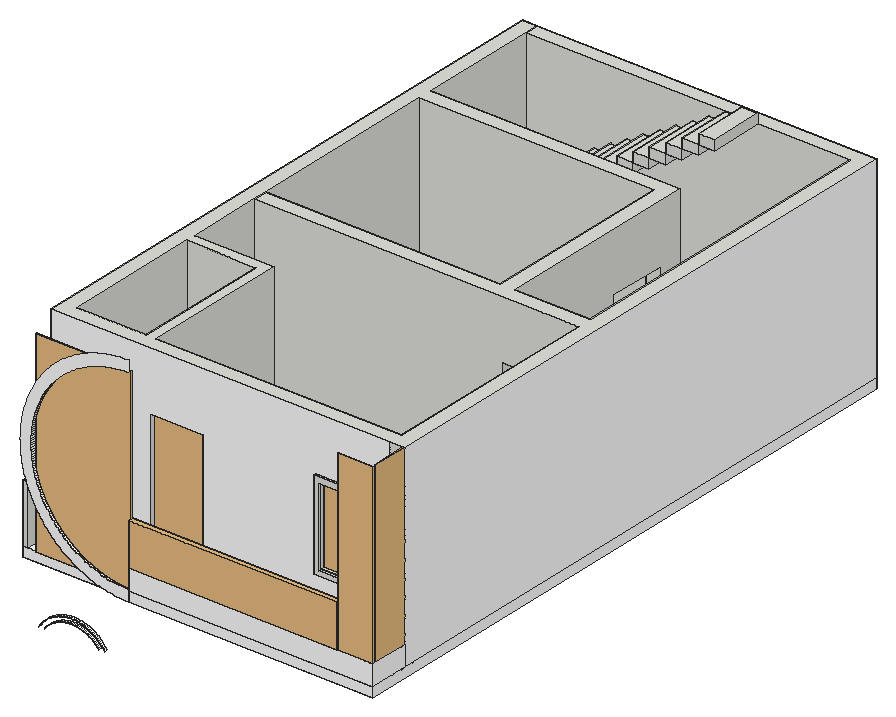
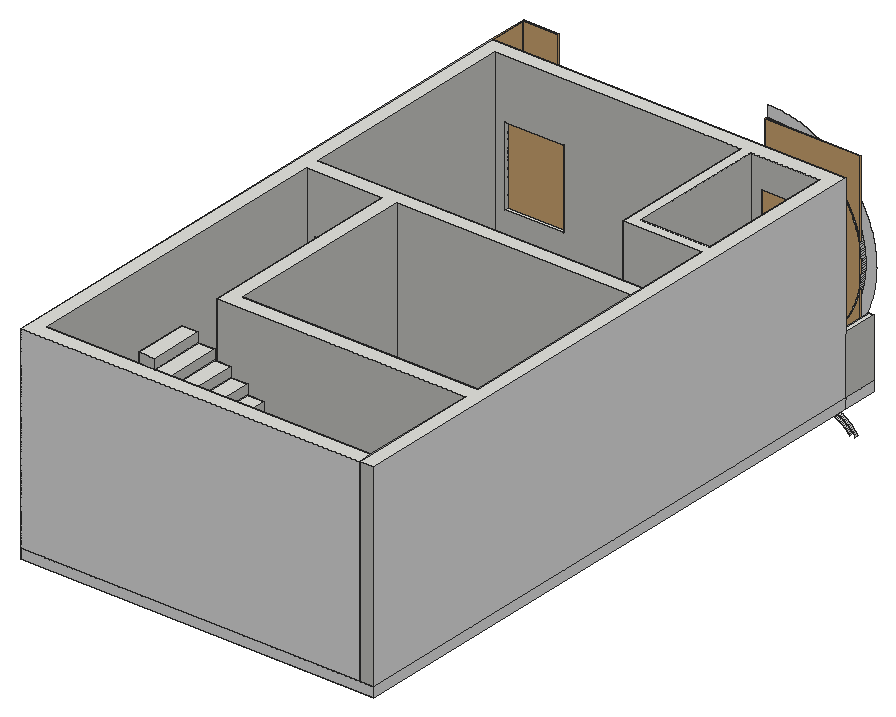
# SketchUp Ruby script. Lengths in inches.
U = 1.inch
M = Sketchup.active_model
def pt(a) = Geom::Point3d.new(a.map { |v| v * U })
def face(e, loops, mat)
  f = e.add_face(loops[0].map { |a| pt(a) })
  loops[1..].each { |l| e.add_face(l.map { |a| pt(a) }).erase! }
  f.material = f.back_material = mat if mat
  f
end
# faces: each face lists its corners as indices into pts; further lists are holes
def faces(e, pts, list, mat = nil) = list.each { |f| face(e, (f[0].is_a?(Array) ? f : [f]).map { |l| l.map { |i| pts[i] } }, mat) }
# xy, xz, yz: faces in a plane at the given z, y or x. An outline is a flat list of corners, or four numbers for a rectangle; further outlines are holes
def ring(l) = l.size == 4 ? [[l[0], l[1]], [l[2], l[1]], [l[2], l[3]], [l[0], l[3]]] : l.each_slice(2).to_a
def flat(e, list, mat, &to3) = list.each { |f| face(e, (f[0].is_a?(Array) ? f : [f]).map { |l| ring(l).map { |u, v| to3.(u, v) } }, mat) }
def xy(e, z, list, mat = nil) = flat(e, list, mat) { |x, y| [x, y, z] }
def xz(e, y, list, mat = nil) = flat(e, list, mat) { |x, z| [x, y, z] }
def yz(e, x, list, mat = nil) = flat(e, list, mat) { |y, z| [x, y, z] }
def lines(e, pts, list) = list.each { |a, b| e.add_line(pt(pts[a]), pt(pts[b])) }
# prism: a flat outline (further loops are holes) pulled along v
def prism(e, loops, v, mat = nil)
  f = face(e, loops, mat); d = Geom::Vector3d.new(v.map { |x| x * U })
  f.pushpull(f.normal.samedirection?(d) ? d.length : -d.length)
end
def box(e, o, s, mat = nil) = prism(e, [[o, [o[0] + s[0], o[1], o[2]], [o[0] + s[0], o[1] + s[1], o[2]], [o[0], o[1] + s[1], o[2]]]], [0, 0, s[2]], mat)
def at(x, y, z, deg = 0) = Geom::Transformation.translation(pt([x, y, z])) * Geom::Transformation.rotation(ORIGIN, Z_AXIS, deg.degrees)
def axes(o, x, y, z) = Geom::Transformation.new([*x, 0, *y, 0, *z, 0, *pt(o).to_a, 1])
def part(name) = M.definitions.add(name)
# library, detail: a bought-in or finely detailed component or shape, given as its bounding box
def library(name, o, s) = part(name).tap { |d| box(d.entities, o, s) }
def detail(e, o, s) = box(e.add_group.entities, o, s)
def put(e, d, t, mat = nil) = e.add_instance(d, t).tap { |i| i.material = mat if mat }
def group(e, t, mat = nil) = e.add_group.tap { |g| g.transformation = t; g.material = mat if mat }.entities
root = M.entities
M.materials.add("Leather White 002 15.0cm").color = [255, 255, 255]
M.materials.add("Manhattan Creative Coating ML 1016B 24.75cm").color = [255, 255, 255]
M.materials.add("Napura - nsi3013 29.32cm").color = [255, 255, 255]
M.materials.add("Wood 012 27.21cm").color = [255, 255, 255]
c1 = library("Door 243 053",[-21.6,-2.79,-0.07],[43.2,5.58,82.64])
c2 = part("Stair tread")
box(c2.entities,[0,0,0],[10,33,6])
c3 = part("Stair landing")
box(c3.entities,[-32,0,0],[42,72,6])
c4 = part("Group\#2")
put(c4.entities,c2,at(82,39,90))
put(c4.entities,c2,at(92,39,96))
put(c4.entities,c2,at(102,39,102))
put(c4.entities,c2,at(72,39,84))
put(c4.entities,c2,at(112,39,108))
put(c4.entities,c2,at(62,39,78))
put(c4.entities,c2,at(122,39,114))
put(c4.entities,c2,at(52,39,72))
put(c4.entities,c2,at(52,0,48))
put(c4.entities,c2,at(42,0,54))
put(c4.entities,c3,at(32,0,60))
put(c4.entities,c2,at(112,0,12))
put(c4.entities,c2,at(122,0,6))
put(c4.entities,c2,at(82,0,30))
put(c4.entities,c2,at(92,0,24))
put(c4.entities,c2,at(72,0,36))
put(c4.entities,c2,at(62,0,42))
put(c4.entities,c2,at(132,0,0))
put(c4.entities,c2,at(102,0,18))
put(c4.entities,c2,at(42,39,66))
put(c4.entities,c2,at(132,39,120))
c5 = part("Group\#14")
box(c5.entities,[0,0,0],[3,21,36])
c6 = library("Group594\#1",[-29.72,-59.43,0],[58,118.86,1])
c7 = library("Group\#13",[0,0,0],[21.6875,1,109.4375])
c8 = library("Group\#17",[0,0,0],[21.6875,1,109.4375])
c9 = library("Group\#15",[0,0,0],[131.45,3.15,25.98])
c10 = library("Window Crafter Sliding",[0,-0.55,0],[36,4.49,48])
c11 = library("Window Crafter Awning",[0,-9.5,0],[24,11.27,18])
xy(root,252,[[66.79,50.93,66.79,53.93,213,53.93,213,74.93,216,74.93,216,50.93]])
xy(root,264.55,[[66.79,50.93,216,50.93,216,74.93,213,74.93,213,53.93,66.79,53.93]])
xz(root,50.93,[[66.79,246,66.79,252.55,65.55,252.56,64.31,252.6,63.0625,252.67,61.82,252.76,60.58,252.88,59.34,253.02,58.11,253.1875,56.88,253.38,55.66,253.6,54.43,253.85,53.22,254.12,52.01,254.42,50.81,254.74,49.61,255.09,48.42,255.46,47.24,255.86,46.07,256.28,44.91,256.73,43.76,257.2,42.62,257.69,41.48,258.21,40.36,258.75,39.25,259.32,38.16,259.9,37.07,260.52,36,261.15,34.94,261.81,33.9,262.48,32.87,263.18,31.85,263.91,30.85,264.65,29.87,265.41,28.9,266.19,27.95,267,27.02,267.82,26.1,268.66,25.2,269.53,24.32,270.41,23.46,271.3,22.62,272.22,21.79,273.16,20.99,274.11,20.21,275.07,19.44,276.06,18.7,277.06,17.98,278.07,17.28,279.1,16.6,280.15,15.94,281.2,15.3125,282.28,14.7,283.36,14.11,284.46,13.55,285.57,13,286.6875,12.49,287.82,11.99,288.96,11.52,290.12,11.07,291.28,10.65,292.45,10.26,293.63,9.88,294.82,9.54,296.01,9.21,297.22,8.92,298.42,8.65,299.64,8.4,300.86,8.18,302.09,7.98,303.32,7.82,304.55,7.67,305.79,7.55,307.03,7.46,308.27,7.4,309.51,7.36,310.76,7.35,312,7.36,313.24,7.4,314.49,7.46,315.73,7.55,316.97,7.67,318.21,7.82,319.45,7.98,320.68,8.18,321.91,8.4,323.14,8.65,324.36,8.92,325.58,9.21,326.78,9.54,327.99,9.88,329.18,10.26,330.37,10.65,331.55,11.07,332.72,11.52,333.88,11.99,335.04,12.49,336.18,13,337.3125,13.55,338.43,14.11,339.54,14.7,340.64,15.3125,341.72,15.94,342.8,16.6,343.85,17.28,344.9,17.98,345.93,18.7,346.94,19.44,347.94,20.21,348.93,20.99,349.89,21.79,350.84,22.62,351.78,23.46,352.7,24.32,353.59,25.2,354.47,26.1,355.34,27.02,356.18,27.95,357,28.9,357.81,29.87,358.59,30.85,359.35,31.85,360.09,32.87,360.82,33.9,361.52,34.94,362.19,36,362.85,37.07,363.48,38.16,364.1,39.25,364.68,40.36,365.25,41.48,365.79,42.62,366.31,43.76,366.8,44.91,367.27,46.07,367.72,47.24,368.14,48.42,368.54,49.61,368.91,50.81,369.26,52.01,369.58,53.22,369.88,54.43,370.15,55.66,370.4,56.88,370.62,58.11,370.8125,59.34,370.98,60.58,371.12,61.82,371.24,63.0625,371.33,64.31,371.4,65.55,371.44,66.79,371.45,66.79,378,65.41,377.99,64.03,377.94,62.65,377.87,61.27,377.77,59.9,377.64,58.52,377.48,57.15,377.29,55.79,377.08,54.43,376.83,53.07,376.56,51.72,376.26,50.38,375.93,49.05,375.57,47.72,375.18,46.4,374.77,45.09,374.33,43.79,373.86,42.5,373.37,41.22,372.84,39.95,372.29,38.69,371.72,37.45,371.12,36.22,370.49,35,369.84,33.79,369.16,32.61,368.45,31.43,367.73,30.27,366.97,29.13,366.2,28,365.4,26.89,364.57,25.8,363.72,24.72,362.85,23.67,361.96,22.63,361.05,21.61,360.11,20.62,359.16,19.64,358.18,18.68,357.18,17.75,356.16,16.83,355.125,15.94,354.07,15.07,353,14.22,351.9,13.4,350.79,12.6,349.67,11.82,348.52,11.07,347.36,10.34,346.19,9.64,345,8.96,343.8,8.31,342.58,7.68,341.35,7.08,340.1,6.5,338.84,5.95,337.58,5.43,336.3,4.93,335.01,4.47,333.71,4.03,332.4,3.61,331.08,3.23,329.75,2.87,328.41,2.54,327.07,2.24,325.72,1.96,324.37,1.72,323.01,1.5,321.64,1.32,320.27,1.16,318.9,1.03,317.52,0.93,316.14,0.85,314.76,0.81,313.38,0.79,312,0.81,310.62,0.85,309.24,0.93,307.86,1.03,306.48,1.16,305.1,1.32,303.73,1.5,302.36,1.72,300.99,1.96,299.63,2.24,298.28,2.54,296.93,2.87,295.59,3.23,294.25,3.61,292.92,4.03,291.6,4.47,290.29,4.93,288.99,5.43,287.7,5.95,286.42,6.5,285.16,7.08,283.9,7.68,282.65,8.31,281.42,8.96,280.2,9.64,279,10.34,277.81,11.07,276.64,11.82,275.48,12.6,274.33,13.4,273.21,14.22,272.1,15.07,271,15.94,269.93,16.83,268.875,17.75,267.84,18.68,266.82,19.64,265.82,20.62,264.84,21.61,263.89,22.63,262.95,23.67,262.04,24.72,261.15,25.8,260.28,26.89,259.43,28,258.6,29.13,257.8,30.27,257.03,31.43,256.27,32.61,255.55,33.79,254.84,35,254.16,36.22,253.51,37.45,252.88,38.69,252.28,39.95,251.71,41.22,251.16,42.5,250.63,43.79,250.14,45.09,249.67,46.4,249.23,47.72,248.82,49.05,248.43,50.38,248.07,51.72,247.74,53.07,247.44,54.43,247.17,55.79,246.92,57.15,246.71,58.52,246.52,59.9,246.36,61.27,246.23,62.65,246.13,64.03,246.06,65.41,246.01]],"Leather White 002 15.0cm")
xz(root,50.93,[[66.79,252,216,264.55]],"Manhattan Creative Coating ML 1016B 24.75cm")
xz(root,53.93,[[66.79,252,213,264.55]])
xz(root,74.93,[[213,252,216,264.55]])
yz(root,66.79,[[50.93,252,53.93,252.55],[50.93,252.55,53.93,264.55]])
yz(root,213,[[53.93,252,74.93,264.55]])
yz(root,216,[[50.93,252,74.93,264.55]],"Manhattan Creative Coating ML 1016B 24.75cm")
p = [[17.08,50.93,214.69],[17.62,50.93,215.38],[17.62,48.93,215.38],[17.08,48.93,214.69],[14.21,50.93,215.61],[13.66,50.93,214.78],
  [13.66,48.93,214.78],[14.21,48.93,215.61],[49.8,50.93,215.55],[50.35,50.93,214.87],[50.35,48.93,214.87],[49.8,48.93,215.55],
  [53.77,50.93,214.98],[53.21,50.93,215.81],[53.21,48.93,215.81],[53.77,48.93,214.98],[18.1875,50.93,216.05],[18.1875,48.93,216.05],
  [49.22,50.93,216.21],[49.22,48.93,216.21],[14.79,50.93,216.42],[14.79,48.93,216.42],[52.62,50.93,216.61],[52.62,48.93,216.61],
  [18.78,50.93,216.6875],[18.78,48.93,216.6875],[48.62,50.93,216.84],[48.62,48.93,216.84],[15.4,50.93,217.2],[15.4,48.93,217.2],
  [52,50.93,217.39],[52,48.93,217.39],[19.41,50.93,217.3],[19.41,48.93,217.3],[47.99,50.93,217.45],[47.99,48.93,217.45],
  [16.05,50.93,217.96],[16.05,48.93,217.96],[20.05,50.93,217.89],[20.05,48.93,217.89],[51.35,50.93,218.14],[51.35,48.93,218.14],
  [47.34,50.93,218.03],[47.34,48.93,218.03],[20.72,50.93,218.45],[20.72,48.93,218.45],[16.72,50.93,218.68],[16.72,48.93,218.68],
  [46.66,50.93,218.59],[46.66,48.93,218.59],[50.66,50.93,218.86],[50.66,48.93,218.86],[21.42,50.93,218.99],[21.42,48.93,218.99],
  [45.96,50.93,219.11],[45.96,48.93,219.11],[17.43,50.93,219.38],[17.43,48.93,219.38],[49.95,50.93,219.55],[49.95,48.93,219.55],
  [22.13,50.93,219.49],[22.13,48.93,219.49],[45.24,50.93,219.61],[45.24,48.93,219.61],[18.17,50.93,220.05],[18.17,48.93,220.05],
  [22.87,50.93,219.96],[22.87,48.93,219.96],[44.5,50.93,220.07],[44.5,48.93,220.07],[49.2,50.93,220.21],[49.2,48.93,220.21],
  [23.625,50.93,220.4],[23.625,48.93,220.4],[18.93,50.93,220.69],[18.93,48.93,220.69],[43.74,50.93,220.5],[43.74,48.93,220.5],
  [48.43,50.93,220.84],[48.43,48.93,220.84],[24.4,50.93,220.8125],[24.4,48.93,220.8125],[42.97,50.93,220.91],[42.97,48.93,220.91],
  [19.72,50.93,221.3],[19.72,48.93,221.3],[25.1875,50.93,221.1875],[25.1875,48.93,221.1875],[47.64,50.93,221.44],[47.64,48.93,221.44],
  [42.17,50.93,221.27],[42.17,48.93,221.27],[25.99,50.93,221.53],[25.99,48.93,221.53],[20.53,50.93,221.87],[20.53,48.93,221.87],
  [41.36,50.93,221.61],[41.36,48.93,221.61],[46.82,50.93,222],[46.82,48.93,222],[26.81,50.93,221.84],[26.81,48.93,221.84],
  [40.54,50.93,221.91],[40.54,48.93,221.91],[27.64,50.93,222.11],[27.64,48.93,222.11],[21.37,50.93,222.41],[21.37,48.93,222.41],
  [39.71,50.93,222.18],[39.71,48.93,222.18],[45.98,50.93,222.53],[45.98,48.93,222.53],[28.48,50.93,222.35],[28.48,48.93,222.35],
  [38.87,50.93,222.41],[38.87,48.93,222.41],[22.23,50.93,222.91],[22.23,48.93,222.91],[29.33,50.93,222.56],[29.33,48.93,222.56],
  [38.01,50.93,222.6],[38.01,48.93,222.6],[45.11,50.93,223.03],[45.11,48.93,223.03],[30.19,50.93,222.73],[30.19,48.93,222.73],
  [37.15,50.93,222.76],[37.15,48.93,222.76],[31.05,50.93,222.86],[31.05,48.93,222.86],[36.29,50.93,222.88],[36.29,48.93,222.88],
  [23.11,50.93,223.375],[23.11,48.93,223.375],[31.92,50.93,222.95],[31.92,48.93,222.95],[35.42,50.93,222.97],[35.42,48.93,222.97],
  [32.8,50.93,223.01],[32.8,48.93,223.01],[33.67,50.93,223.04],[33.67,48.93,223.04],[34.55,50.93,223.02],[34.55,48.93,223.02],
  [44.23,50.93,223.48],[44.23,48.93,223.48],[24.01,50.93,223.8],[24.01,48.93,223.8],[43.33,50.93,223.9],[43.33,48.93,223.9],
  [24.92,50.93,224.19],[24.92,48.93,224.19],[42.41,50.93,224.28],[42.41,48.93,224.28],[25.85,50.93,224.54],[25.85,48.93,224.54],
  [41.47,50.93,224.625],[41.47,48.93,224.625],[26.8,50.93,224.86],[26.8,48.93,224.86],[40.53,50.93,224.93],[40.53,48.93,224.93],
  [27.75,50.93,225.13],[27.75,48.93,225.13],[39.57,50.93,225.1875],[39.57,48.93,225.1875],[28.72,50.93,225.36],[28.72,48.93,225.36],
  [38.6,50.93,225.41],[38.6,48.93,225.41],[29.7,50.93,225.55],[29.7,48.93,225.55],[37.62,50.93,225.59],[37.62,48.93,225.59],
  [30.68,50.93,225.7],[30.68,48.93,225.7],[36.63,50.93,225.73],[36.63,48.93,225.73],[31.67,50.93,225.8125],[31.67,48.93,225.8125],
  [35.64,50.93,225.83],[35.64,48.93,225.83],[32.66,50.93,225.88],[32.66,48.93,225.88],[34.65,50.93,225.89],[34.65,48.93,225.89],
  [33.66,50.93,225.91],[33.66,48.93,225.91],[63.0625,50.93,252.67],[64.31,50.93,252.6],[64.31,53.93,252.6],[63.0625,53.93,252.67],
  [65.55,50.93,252.56],[65.55,53.93,252.56],[66.79,50.93,252.55],[66.79,53.93,252.55],[61.82,50.93,252.76],[61.82,53.93,252.76],
  [60.58,50.93,252.88],[60.58,53.93,252.88],[59.34,50.93,253.02],[59.34,53.93,253.02],[58.11,50.93,253.1875],[58.11,53.93,253.1875],
  [56.88,50.93,253.38],[56.88,53.93,253.38],[55.66,50.93,253.6],[55.66,53.93,253.6],[54.43,50.93,253.85],[54.43,53.93,253.85],
  [53.22,50.93,254.12],[53.22,53.93,254.12],[52.01,50.93,254.42],[52.01,53.93,254.42],[50.81,50.93,254.74],[50.81,53.93,254.74],
  [49.61,50.93,255.09],[49.61,53.93,255.09],[48.42,50.93,255.46],[48.42,53.93,255.46],[47.24,50.93,255.86],[47.24,53.93,255.86],
  [46.07,50.93,256.28],[46.07,53.93,256.28],[44.91,50.93,256.73],[44.91,53.93,256.73],[43.76,50.93,257.2],[43.76,53.93,257.2],
  [42.62,50.93,257.69],[42.62,53.93,257.69],[41.48,50.93,258.21],[41.48,53.93,258.21],[40.36,50.93,258.75],[40.36,53.93,258.75],
  [39.25,50.93,259.32],[39.25,53.93,259.32],[38.16,50.93,259.9],[38.16,53.93,259.9],[37.07,50.93,260.52],[37.07,53.93,260.52],
  [36,50.93,261.15],[36,53.93,261.15],[34.94,50.93,261.81],[34.94,53.93,261.81],[33.9,50.93,262.48],[33.9,53.93,262.48],
  [32.87,50.93,263.18],[32.87,53.93,263.18],[31.85,50.93,263.91],[31.85,53.93,263.91],[30.85,50.93,264.65],[30.85,53.93,264.65],
  [29.87,50.93,265.41],[29.87,53.93,265.41],[28.9,50.93,266.19],[28.9,53.93,266.19],[27.95,50.93,267],[27.95,53.93,267],
  [27.02,50.93,267.82],[27.02,53.93,267.82],[26.1,50.93,268.66],[26.1,53.93,268.66],[25.2,50.93,269.53],[25.2,53.93,269.53],
  [24.32,50.93,270.41],[24.32,53.93,270.41],[23.46,50.93,271.3],[23.46,53.93,271.3],[22.62,50.93,272.22],[22.62,53.93,272.22],
  [21.79,50.93,273.16],[21.79,53.93,273.16],[20.99,50.93,274.11],[20.99,53.93,274.11],[20.21,50.93,275.07],[20.21,53.93,275.07],
  [19.44,50.93,276.06],[19.44,53.93,276.06],[18.7,50.93,277.06],[18.7,53.93,277.06],[17.98,50.93,278.07],[17.98,53.93,278.07],
  [17.28,50.93,279.1],[17.28,53.93,279.1],[16.6,50.93,280.15],[16.6,53.93,280.15],[15.94,50.93,281.2],[15.94,53.93,281.2],
  [15.3125,50.93,282.28],[15.3125,53.93,282.28],[14.7,50.93,283.36],[14.7,53.93,283.36],[14.11,50.93,284.46],[14.11,53.93,284.46],
  [13.55,50.93,285.57],[13.55,53.93,285.57],[13,50.93,286.6875],[13,53.93,286.6875],[12.49,50.93,287.82],[12.49,53.93,287.82],
  [11.99,50.93,288.96],[11.99,53.93,288.96],[11.52,50.93,290.12],[11.52,53.93,290.12],[11.07,50.93,291.28],[11.07,53.93,291.28],
  [10.65,50.93,292.45],[10.65,53.93,292.45],[10.26,50.93,293.63],[10.26,53.93,293.63],[9.88,50.93,294.82],[9.88,53.93,294.82],
  [9.54,50.93,296.01],[9.54,53.93,296.01],[9.21,50.93,297.22],[9.21,53.93,297.22],[8.92,50.93,298.42],[8.92,53.93,298.42],
  [8.65,50.93,299.64],[8.65,53.93,299.64],[8.4,50.93,300.86],[8.4,53.93,300.86],[8.18,50.93,302.09],[8.18,53.93,302.09],
  [7.98,50.93,303.32],[7.98,53.93,303.32],[7.82,50.93,304.55],[7.82,53.93,304.55],[7.67,50.93,305.79],[7.67,53.93,305.79],
  [7.55,50.93,307.03],[7.55,53.93,307.03],[7.46,50.93,308.27],[7.46,53.93,308.27],[7.4,50.93,309.51],[7.4,53.93,309.51],
  [7.36,50.93,310.76],[7.36,53.93,310.76],[7.35,50.93,312],[7.35,53.93,312],[7.36,50.93,313.24],[7.36,53.93,313.24],
  [7.4,50.93,314.49],[7.4,53.93,314.49],[7.46,50.93,315.73],[7.46,53.93,315.73],[7.55,50.93,316.97],[7.55,53.93,316.97],
  [7.67,50.93,318.21],[7.67,53.93,318.21],[7.82,50.93,319.45],[7.82,53.93,319.45],[7.98,50.93,320.68],[7.98,53.93,320.68],
  [8.18,50.93,321.91],[8.18,53.93,321.91],[8.4,50.93,323.14],[8.4,53.93,323.14],[8.65,50.93,324.36],[8.65,53.93,324.36],
  [8.92,50.93,325.58],[8.92,53.93,325.58],[9.21,50.93,326.78],[9.21,53.93,326.78],[9.54,50.93,327.99],[9.54,53.93,327.99],
  [9.88,50.93,329.18],[9.88,53.93,329.18],[10.26,50.93,330.37],[10.26,53.93,330.37],[10.65,50.93,331.55],[10.65,53.93,331.55],
  [11.07,50.93,332.72],[11.07,53.93,332.72],[11.52,50.93,333.88],[11.52,53.93,333.88],[11.99,50.93,335.04],[11.99,53.93,335.04],
  [12.49,50.93,336.18],[12.49,53.93,336.18],[13,50.93,337.3125],[13,53.93,337.3125],[13.55,50.93,338.43],[13.55,53.93,338.43],
  [14.11,50.93,339.54],[14.11,53.93,339.54],[14.7,50.93,340.64],[14.7,53.93,340.64],[15.3125,50.93,341.72],[15.3125,53.93,341.72],
  [15.94,50.93,342.8],[15.94,53.93,342.8],[16.6,50.93,343.85],[16.6,53.93,343.85],[17.28,50.93,344.9],[17.28,53.93,344.9],
  [17.98,50.93,345.93],[17.98,53.93,345.93],[18.7,50.93,346.94],[18.7,53.93,346.94],[19.44,50.93,347.94],[19.44,53.93,347.94],
  [20.21,50.93,348.93],[20.21,53.93,348.93]]
faces(root,p,[[0,1,2,3],[4,5,6,7],[8,9,10,11],[12,13,14,15],[1,16,17,2],[18,8,11,19],[20,4,7,21],[13,22,23,14],
  [16,24,25,17],[26,18,19,27],[28,20,21,29],[22,30,31,23],[24,32,33,25],[34,26,27,35],[36,28,29,37],[32,38,39,33],
  [30,40,41,31],[42,34,35,43],[38,44,45,39],[46,36,37,47],[48,42,43,49],[40,50,51,41],[44,52,53,45],[54,48,49,55],
  [56,46,47,57],[50,58,59,51],[52,60,61,53],[62,54,55,63],[64,56,57,65],[60,66,67,61],[68,62,63,69],[58,70,71,59],
  [66,72,73,67],[74,64,65,75],[76,68,69,77],[70,78,79,71],[72,80,81,73],[82,76,77,83],[84,74,75,85],[80,86,87,81],
  [78,88,89,79],[90,82,83,91],[86,92,93,87],[94,84,85,95],[96,90,91,97],[88,98,99,89],[92,100,101,93],[102,96,97,103],
  [100,104,105,101],[106,94,95,107],[108,102,103,109],[98,110,111,99],[104,112,113,105],[114,108,109,115],[116,106,107,117],[112,118,119,113],
  [120,114,115,121],[110,122,123,111],[118,124,125,119],[126,120,121,127],[124,128,129,125],[130,126,127,131],[132,116,117,133],[128,134,135,129],
  [136,130,131,137],[134,138,139,135],[138,140,141,139],[140,142,143,141],[142,136,137,143],[122,144,145,123],[146,132,133,147],[144,148,149,145],
  [150,146,147,151],[148,152,153,149],[154,150,151,155],[152,156,157,153],[158,154,155,159],[156,160,161,157],[162,158,159,163],[160,164,165,161],
  [166,162,163,167],[164,168,169,165],[170,166,167,171],[168,172,173,169],[174,170,171,175],[172,176,177,173],[178,174,175,179],[176,180,181,177],
  [182,178,179,183],[180,184,185,181],[186,182,183,187],[184,186,187,185],[188,189,190,191],[189,192,193,190],[192,194,195,193],[196,188,191,197],
  [198,196,197,199],[200,198,199,201],[202,200,201,203],[204,202,203,205],[206,204,205,207],[208,206,207,209],[210,208,209,211],[212,210,211,213],
  [214,212,213,215],[216,214,215,217],[218,216,217,219],[220,218,219,221],[222,220,221,223],[224,222,223,225],[226,224,225,227],[228,226,227,229],
  [230,228,229,231],[232,230,231,233],[234,232,233,235],[236,234,235,237],[238,236,237,239],[240,238,239,241],[242,240,241,243],[244,242,243,245],
  [246,244,245,247],[248,246,247,249],[250,248,249,251],[252,250,251,253],[254,252,253,255],[256,254,255,257],[258,256,257,259],[260,258,259,261],
  [262,260,261,263],[264,262,263,265],[266,264,265,267],[268,266,267,269],[270,268,269,271],[272,270,271,273],[274,272,273,275],[276,274,275,277],
  [278,276,277,279],[280,278,279,281],[282,280,281,283],[284,282,283,285],[286,284,285,287],[288,286,287,289],[290,288,289,291],[292,290,291,293],
  [294,292,293,295],[296,294,295,297],[298,296,297,299],[300,298,299,301],[302,300,301,303],[304,302,303,305],[306,304,305,307],[308,306,307,309],
  [310,308,309,311],[312,310,311,313],[314,312,313,315],[316,314,315,317],[318,316,317,319],[320,318,319,321],[322,320,321,323],[324,322,323,325],
  [326,324,325,327],[328,326,327,329],[330,328,329,331],[332,330,331,333],[334,332,333,335],[336,334,335,337],[338,336,337,339],[340,338,339,341],
  [342,340,341,343],[344,342,343,345],[346,344,345,347],[348,346,347,349],[350,348,349,351],[352,350,351,353],[354,352,353,355],[356,354,355,357],
  [358,356,357,359],[360,358,359,361],[362,360,361,363],[364,362,363,365],[366,364,365,367],[368,366,367,369],[370,368,369,371],[372,370,371,373],
  [374,372,373,375],[376,374,375,377],[378,376,377,379],[380,378,379,381],[382,380,381,383],[384,382,383,385],[386,384,385,387],[388,386,387,389],
  [390,388,389,391],[392,390,391,393],[394,392,393,395],[396,394,395,397],[398,396,397,399],[400,398,399,401],[402,400,401,403]],"Leather White 002 15.0cm")
g1 = group(root,at(0,74.93,246),"Manhattan Creative Coating ML 1016B 24.75cm")
prism(g1,[[[216,360,0],[216,-24,0],[66.79,-24,0],[66.79,-21,0],[0,-21,0],[0,0,0],[0,360,0]],[[151,279,0],[151,351,0],[9,351,0],[9,279,0]]],[0,0,6])
put(root,c1,axes([76.96,79.6875,252],[0.7407,0,0],[0,1,0],[0,0,1.02907]))
g2 = group(root,at(0,74.93,252))
xy(g2,0,[[0,0,0,360,9,360,9,279.04,161.02,279.04,161.02,264,152,264,152,270.04,9,270.04,9,99,13,99,13,93,9,93,9,0],[9,0,9,9,51.2,9,51.2,93,44.96,93,44.96,99,57.2,99,57.2,9,61.2,9,61.2,0],[9,144,9,153,152,153,152,228,161.02,228,161.02,144],[201.62,144,207,153],[9,351,207,360]])
xy(g2,36,[[165.0625,0,201.0625,9]])
xy(g2,84,[[20,0,44,9],[61.2,0,93.17,9],[165.0625,0,201.0625,9],[13,93,44.96,99],[161.02,144,201.62,153],
  [152,228,161.02,264]])
xy(g2,102,[[20,0,44,9]])
xy(g2,120,[[[0,0,207,0,207,9,57.2,9,57.2,99,9,99,9,270.04,152,270.04,152,153,9,153,9,144,207,144,207,0,216,0,216,360,9,360,9,351,207,351,207,153,161.02,153,161.02,279.04,9,279.04,9,360,0,360],[9,9,51.2,93]]])
xz(g2,0,[[207,0,216,120]])
xz(g2,0,[[[0,0,61.2,0,61.2,84,93.17,84,93.17,0,207,0,207,120,0,120],[165.0625,36,201.0625,84],[20,84,44,102]]],"Napura - nsi3013 29.32cm")
xz(g2,9,[[[9,0,51.2,120],[20,84,44,102]],[[57.2,0,57.2,120,207,120,207,0,93.17,0,93.17,84,61.2,84,61.2,0],[165.0625,36,201.0625,84]]])
xz(g2,93,[[9,0,13,0,13,84,44.96,84,44.96,0,51.2,0,51.2,120,9,120]])
xz(g2,99,[[9,0,9,120,57.2,120,57.2,0,44.96,0,44.96,84,13,84,13,0]])
xz(g2,144,[[9,0,161.02,0,161.02,84,201.62,84,201.62,0,207,0,207,120,9,120]])
xz(g2,153,[[9,0,152,120],[201.62,0,201.62,84,161.02,84,161.02,120,207,120,207,0]])
xz(g2,228,[[152,0,161.02,84]])
xz(g2,264,[[152,0,161.02,84]])
xz(g2,270.04,[[9,0,152,120]])
xz(g2,279.04,[[9,0,161.02,120]])
xz(g2,351,[[9,0,207,120]])
xz(g2,360,[[0,0,9,120]])
xz(g2,360,[[9,0,216,120]],"Napura - nsi3013 29.32cm")
yz(g2,0,[[0,0,360,120]],"Napura - nsi3013 29.32cm")
yz(g2,9,[[9,0,93,120],[99,0,144,120],[144,0,153,120],[153,0,270.04,120],[279.04,0,351,120],
  [351,0,360,120]])
yz(g2,13,[[93,0,99,84]])
yz(g2,20,[[0,84,9,102]])
yz(g2,44,[[0,84,9,102]])
yz(g2,44.96,[[93,0,99,84]])
yz(g2,51.2,[[9,0,93,120]])
yz(g2,57.2,[[9,0,99,120]])
yz(g2,61.2,[[0,0,9,84]])
yz(g2,93.17,[[0,0,9,84]])
yz(g2,152,[[153,0,153,120,270.04,120,270.04,0,264,0,264,84,228,84,228,0]])
yz(g2,161.02,[[144,0,228,0,228,84,264,84,264,0,279.04,0,279.04,120,153,120,153,84,144,84]])
yz(g2,165.0625,[[0,36,9,84]])
yz(g2,201.0625,[[0,36,9,84]])
yz(g2,201.62,[[144,0,153,84]])
yz(g2,207,[[9,0,144,120],[153,0,351,120]])
yz(g2,216,[[0,0,360,120]],"Napura - nsi3013 29.32cm")
put(root,c4,at(9,353.93,252))
put(root,c5,at(0,53.93,252))
put(root,c6,axes([38.52,53.43,311.98],[1,0,0],[0,0,1],[0,-1,0]),"Wood 012 27.21cm")
put(root,c7,axes([194.3125,50.9375,264.55],[1,0,0],[0,1,0],[0,0,0.98183]))
put(root,c8,axes([216,53.24,264.55],[0,1,0],[-1,0,0],[0,0,0.98183]))
put(root,c9,axes([66.79,50.86,264.55],[0.97005,0,0],[0,1,0],[0,0,1]))
g3 = group(root,at(162.0625,72.93,285))
prism(g3,[[[42,2,0],[0,2,0],[0,2,54],[42,2,54]],[[39,2,51],[3,2,51],[3,2,3],[39,2,3]]],[0,-2,0])
put(root,c10,at(165.0625,77.74,288))
put(root,c11,at(20,82.23,336))
